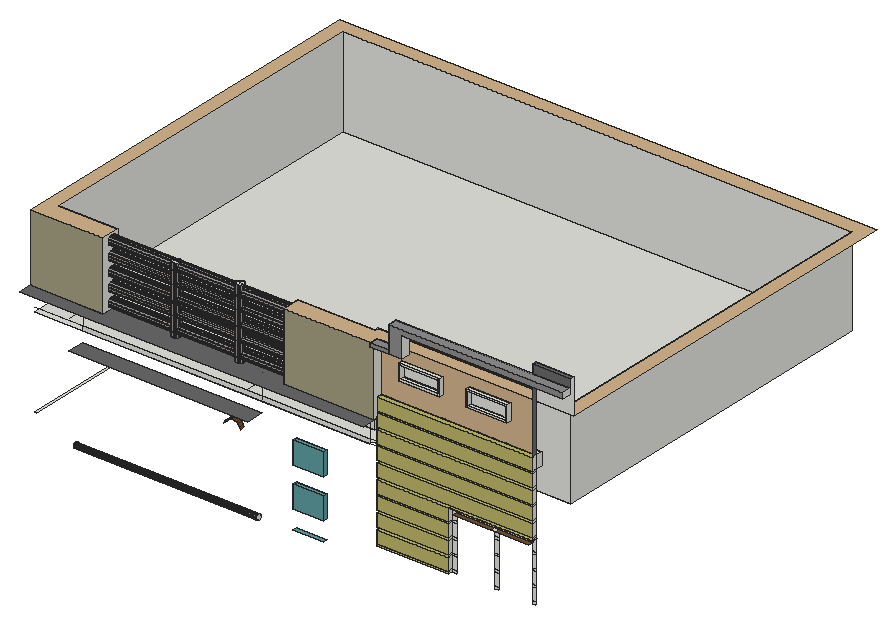
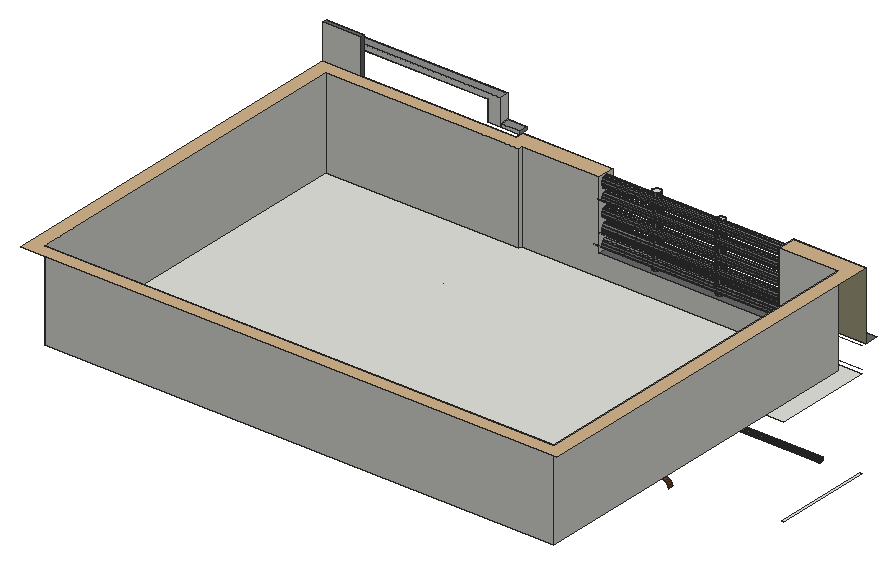
# SketchUp Ruby script. Lengths in inches.
U = 1.inch
M = Sketchup.active_model
def pt(a) = Geom::Point3d.new(a.map { |v| v * U })
def face(e, loops, mat)
  f = e.add_face(loops[0].map { |a| pt(a) })
  loops[1..].each { |l| e.add_face(l.map { |a| pt(a) }).erase! }
  f.material = f.back_material = mat if mat
  f
end
# faces: each face lists its corners as indices into pts; further lists are holes
def faces(e, pts, list, mat = nil) = list.each { |f| face(e, (f[0].is_a?(Array) ? f : [f]).map { |l| l.map { |i| pts[i] } }, mat) }
# xy, xz, yz: faces in a plane at the given z, y or x. An outline is a flat list of corners, or four numbers for a rectangle; further outlines are holes
def ring(l) = l.size == 4 ? [[l[0], l[1]], [l[2], l[1]], [l[2], l[3]], [l[0], l[3]]] : l.each_slice(2).to_a
def flat(e, list, mat, &to3) = list.each { |f| face(e, (f[0].is_a?(Array) ? f : [f]).map { |l| ring(l).map { |u, v| to3.(u, v) } }, mat) }
def xy(e, z, list, mat = nil) = flat(e, list, mat) { |x, y| [x, y, z] }
def xz(e, y, list, mat = nil) = flat(e, list, mat) { |x, z| [x, y, z] }
def yz(e, x, list, mat = nil) = flat(e, list, mat) { |y, z| [x, y, z] }
def lines(e, pts, list) = list.each { |a, b| e.add_line(pt(pts[a]), pt(pts[b])) }
# prism: a flat outline (further loops are holes) pulled along v
def prism(e, loops, v, mat = nil)
  f = face(e, loops, mat); d = Geom::Vector3d.new(v.map { |x| x * U })
  f.pushpull(f.normal.samedirection?(d) ? d.length : -d.length)
end
def box(e, o, s, mat = nil) = prism(e, [[o, [o[0] + s[0], o[1], o[2]], [o[0] + s[0], o[1] + s[1], o[2]], [o[0], o[1] + s[1], o[2]]]], [0, 0, s[2]], mat)
def at(x, y, z, deg = 0) = Geom::Transformation.translation(pt([x, y, z])) * Geom::Transformation.rotation(ORIGIN, Z_AXIS, deg.degrees)
def axes(o, x, y, z) = Geom::Transformation.new([*x, 0, *y, 0, *z, 0, *pt(o).to_a, 1])
def part(name) = M.definitions.add(name)
# library, detail: a bought-in or finely detailed component or shape, given as its bounding box
def library(name, o, s) = part(name).tap { |d| box(d.entities, o, s) }
def detail(e, o, s) = box(e.add_group.entities, o, s)
def put(e, d, t, mat = nil) = e.add_instance(d, t).tap { |i| i.material = mat if mat }
def group(e, t, mat = nil) = e.add_group.tap { |g| g.transformation = t; g.material = mat if mat }.entities
root = M.entities
M.materials.add("[0035_Tan]").color = [210, 180, 140]
M.materials.add("[0057_DarkKhaki]").color = [189, 183, 107]
M.materials.add("[0081_CadetBlue]").color = [95, 158, 160]
M.materials.add("[0134_DimGray]").color = [105, 105, 105]
M.materials.add("[Color M04]").color = [142, 142, 142]
M.materials.add("[Concrete Aggregate Smoke]").color = [154, 150, 148]
M.materials.add("[Sandstone]").color = [118, 81, 52]
M.materials.add("[Stone Coursed Rough]").color = [165, 160, 130]
M.materials.add("[Wood Veneer 01]").color = [120, 70, 37]
xy(root,183.125,[[0,109.375,1.6875,174.625]])
xy(root,183.41,[[230.5,108.71,278.53,111.71]],"[0057_DarkKhaki]")
xy(root,183.75,[[185.74,94.375,206.18,97.375]],"[0081_CadetBlue]")
xy(root,184.9375,[[230.5,108.71,278.53,111.71]],"[0057_DarkKhaki]")
xy(root,193.41,[[230.5,108.71,278.53,111.71]],"[0057_DarkKhaki]")
xy(root,194.9375,[[230.5,108.71,278.53,111.71]],"[0057_DarkKhaki]")
xy(root,196.125,[[185.74,94.375,206.18,97.375]],"[0081_CadetBlue]")
xy(root,203.41,[[230.5,108.71,278.53,111.71]],"[0057_DarkKhaki]")
xy(root,204,[[75.42,171.625,105.42,174.625]],"[Wood Veneer 01]")
xy(root,204.9375,[[230.5,108.71,278.53,111.71]],"[0057_DarkKhaki]")
xy(root,207,[[72.42,171.625,108.42,174.625]],"[Wood Veneer 01]")
xy(root,211.125,[[185.74,94.375,206.18,97.375]],"[0081_CadetBlue]")
xy(root,213.41,[[230.5,108.71,278.53,111.71]],"[0057_DarkKhaki]")
xy(root,214.9375,[[230.5,108.71,278.53,111.71]],"[0057_DarkKhaki]")
xy(root,220.14,[[307.0625,108.71,310.13,111.71]])
xy(root,220.14,[[281.53,108.71,307.0625,111.71],[310.13,108.71,332.6,111.71]],"[Sandstone]")
xy(root,222.6875,[[185.74,94.375,206.18,97.375]],"[0081_CadetBlue]")
xy(root,223.14,[[278.53,108.71,334.9375,111.71],[334.9375,108.71,335.6,111.71]])
xy(root,223.41,[[230.5,108.71,334.9375,111.71]],"[0057_DarkKhaki]")
xy(root,224.9375,[[230.5,108.71,334.9375,111.71]],"[0057_DarkKhaki]")
xy(root,233.41,[[230.5,108.71,334.9375,111.71]],"[0057_DarkKhaki]")
xy(root,234.9375,[[230.5,108.71,334.9375,111.71]],"[0057_DarkKhaki]")
xy(root,236.11,[[32.625,97.375,152.93,109.375]],"[0134_DimGray]")
xy(root,237.6875,[[185.74,94.375,206.18,97.375]],"[0081_CadetBlue]")
xy(root,243,[[0,109.375,0,174.625,228.875,174.625,228.875,111.71,225.1875,111.71,225.1875,109.375]])
xy(root,243.41,[[230.5,108.71,334.9375,111.71]],"[0057_DarkKhaki]")
xy(root,244.9375,[[230.5,108.71,334.9375,111.71]],"[0057_DarkKhaki]")
xy(root,246,[[9,118.375,221.5,118.375,221.5,120.71,351,120.71,351,357,9,357]])
xy(root,253.41,[[230.5,108.71,334.9375,111.71]],"[0057_DarkKhaki]")
xy(root,254.9375,[[230.5,108.71,334.9375,111.71]],"[0057_DarkKhaki]")
xy(root,260.3125,[[32.625,106.375,48.47,109.375],[169.54,106.375,225.1875,109.375],[225.1875,106.375,230.5,109.375],[93.22,109.28,93.6,109.375,92.22,109.375,92.51,109.29]])
xy(root,260.3125,[[[0,97.375,230.5,97.375,230.5,106.375,169.54,106.375,169.54,118.375,48.47,118.375,48.47,106.375,0,106.375],[93.22,109.28,92.51,109.29,92.22,109.375,91.82,109.49,91.2,109.86,90.7,110.38,90.35,111.01,90.18,111.7,90.19,112.42,90.39,113.11,90.76,113.73,91.28,114.22,91.91,114.57,92.6,114.75,93.32,114.73,94.01,114.53,94.625,114.16,95.125,113.65,95.47,113.02,95.65,112.32,95.63,111.61,95.43,110.92,95.06,110.3,94.55,109.8,93.92,109.45,93.6,109.375],[135.16,109.375,134.75,109.49,134.14,109.86,133.64,110.38,133.29,111.01,133.12,111.7,133.13,112.42,133.33,113.11,133.7,113.73,134.22,114.22,134.84,114.57,135.54,114.75,136.26,114.73,136.95,114.53,137.5625,114.16,138.0625,113.65,138.41,113.02,138.58,112.32,138.57,111.61,138.37,110.92,138,110.3,137.49,109.8,136.86,109.45,136.54,109.375]]],"[0134_DimGray]")
xy(root,263.41,[[230.5,108.71,334.9375,111.71]],"[0057_DarkKhaki]")
xy(root,264.9375,[[230.5,111.71,334.9375,116.15]])
xy(root,264.9375,[[230.5,108.71,334.9375,111.71]],"[0057_DarkKhaki]")
xy(root,273.41,[[230.5,111.71,334.9375,116.15]])
xy(root,273.41,[[230.5,108.71,334.9375,111.71]],"[0057_DarkKhaki]")
xy(root,288.05,[[245,108.71,272.5625,111.71],[290.25,108.71,317.8125,111.71]])
xy(root,288.97,[[291.17,108.71,316.89,111.71]])
xy(root,289.17,[[246.12,108.71,271.44,111.71]])
xy(root,297.62,[[246.12,108.71,271.44,111.71]])
xy(root,297.82,[[291.17,108.71,316.89,111.71]])
xy(root,298.74,[[245,108.71,272.5625,111.71],[290.25,108.71,317.8125,111.71]])
xy(root,305.12,[[92.22,109.375,93.6,109.375,93.92,109.45,94.55,109.8,95.06,110.3,95.43,110.92,95.63,111.61,95.65,112.32,95.63,112.38,90.19,112.38,90.18,111.7,90.35,111.01,90.7,110.38,91.2,109.86,91.82,109.49],[90.19,112.38,95.63,112.38,95.47,113.02,95.125,113.65,94.72,114.07,91.11,114.07,90.76,113.73,90.39,113.11,90.19,112.42],[91.11,114.07,94.72,114.07,94.625,114.16,94.01,114.53,93.32,114.73,92.6,114.75,91.91,114.57,91.28,114.22]])
xy(root,306,[[230.5,102.71,243,108.71],[243,102.71,251.83,108.71]])
xy(root,306,[[0,106.375,48.47,106.375,48.47,118.375,9,118.375,9,357,351,357,351,120.71,221.5,120.71,221.5,118.375,169.54,118.375,169.54,106.375,230.5,106.375,230.5,111.71,360,111.71,360,366,0,366]],"[0035_Tan]")
xy(root,306.9375,[[135.16,109.375,136.54,109.375,136.86,109.45,137.49,109.8,138,110.3,138.37,110.92,138.57,111.61,138.58,112.32,138.41,113.02,138.0625,113.65,137.5625,114.16,136.95,114.53,136.26,114.73,135.54,114.75,134.84,114.57,134.22,114.22,133.7,113.73,133.33,113.11,133.13,112.42,133.12,111.7,133.29,111.01,133.64,110.38,134.14,109.86,134.75,109.49]])
xy(root,308.21,[[230.5,102.71,243,108.71]],"[Color M04]")
xy(root,320.08,[[251.83,102.71,360,108.71]])
xy(root,323.78,[[243,102.71,360,108.71]],"[Color M04]")
xy(root,329.5,[[334.9375,108.71,360,111.71]],"[0134_DimGray]")
xz(root,94.375,[[185.74,196.125,206.18,211.125],[185.74,222.6875,206.18,237.6875]],"[0081_CadetBlue]")
xz(root,97.375,[[185.74,196.125,206.18,211.125],[185.74,222.6875,206.18,237.6875]])
xz(root,102.71,[[230.5,306,243,308.21],[243,306,251.83,306,251.83,320.08,360,320.08,360,323.78,243,323.78]],"[Color M04]")
xz(root,106.375,[[0,260.3125,48.47,306],[169.54,260.3125,230.5,306]],"[Stone Coursed Rough]")
xz(root,108.71,[[[245,288.05,272.5625,298.74],[246.12,289.17,271.44,297.62]],[[290.25,288.05,317.8125,298.74],[291.17,288.97,316.89,297.82]],[230.5,306,243,308.21],[243,306,243,323.78,334.9375,323.78,334.9375,320.08,251.83,320.08,251.83,306],[334.9375,320.08,360,323.78]])
xz(root,108.71,[[230.5,184.9375,278.53,193.41],[230.5,194.9375,278.53,203.41],[230.5,204.9375,278.53,213.41],[230.5,214.9375,278.53,214.9375,278.53,223.14,334.9375,223.14,334.9375,223.41,230.5,223.41],[230.5,224.9375,334.9375,233.41],
  [230.5,234.9375,334.9375,243.41],[230.5,244.9375,334.9375,253.41],[230.5,254.9375,334.9375,263.41],[230.5,264.9375,334.9375,273.41]],"[0057_DarkKhaki]")
xz(root,108.71,[[334.9375,323.78,360,329.5]],"[0134_DimGray]")
xz(root,109.375,[[32.625,243,152.93,246],[152.93,243,225.1875,246]])
xz(root,109.375,[[92.22,260.3125,93.6,305.12],[135.16,260.3125,136.54,306.9375]],"[Concrete Aggregate Smoke]")
xz(root,111.71,[[230.5,183.41,278.53,184.9375],[278.53,183.41,281.53,184.9375],[307.0625,183.41,310.13,184.9375],[332.6,183.41,334.9375,184.9375],[230.5,184.9375,278.53,193.41],
  [278.53,184.9375,281.53,193.41],[307.0625,184.9375,310.13,193.41],[332.6,184.9375,334.9375,193.41],[230.5,193.41,278.53,194.9375],[278.53,193.41,281.53,194.9375],
  [307.0625,193.41,310.13,194.9375],[332.6,193.41,334.9375,194.9375],[230.5,194.9375,278.53,203.41],[278.53,194.9375,281.53,203.41],[307.0625,194.9375,310.13,203.41],
  [332.6,194.9375,334.9375,203.41],[230.5,203.41,278.53,204.9375],[278.53,203.41,281.53,204.9375],[307.0625,203.41,310.13,204.9375],[332.6,203.41,334.9375,204.9375],
  [230.5,204.9375,278.53,213.41],[278.53,204.9375,281.53,213.41],[307.0625,204.9375,310.13,213.41],[332.6,204.9375,334.9375,213.41],[230.5,213.41,278.53,214.9375],
  [278.53,213.41,281.53,214.9375],[307.0625,213.41,310.13,214.9375],[332.6,213.41,334.9375,214.9375],[230.5,214.9375,230.5,223.41,334.9375,223.41,334.9375,223.14,278.53,223.14,278.53,214.9375],[278.53,214.9375,281.53,214.9375,281.53,220.14,332.6,220.14,332.6,214.9375,334.9375,214.9375,334.9375,223.14,278.53,223.14],
  [307.0625,214.9375,310.13,220.14],[230.5,224.9375,334.9375,233.41],[230.5,234.9375,334.9375,243.41],[230.5,244.9375,334.9375,253.41],[230.5,254.9375,334.9375,263.41],
  [230.5,264.9375,334.9375,273.41],[[245,288.05,272.5625,298.74],[246.12,289.17,271.44,297.62]],[[290.25,288.05,317.8125,298.74],[291.17,288.97,316.89,297.82]],[291.17,288.97,316.89,297.82],[246.12,289.17,271.44,297.62],
  [334.9375,306,360,329.5]])
xz(root,111.71,[[[230.5,273.41,334.9375,306],[245,288.05,272.5625,298.74],[290.25,288.05,317.8125,298.74]]],"[0035_Tan]")
xz(root,111.71,[[230.5,223.41,334.9375,224.9375],[230.5,233.41,334.9375,234.9375],[230.5,243.41,334.9375,244.9375],[230.5,253.41,334.9375,254.9375],[230.5,263.41,334.9375,264.9375]],"[0057_DarkKhaki]")
xz(root,116.15,[[230.5,264.9375,334.9375,273.41]])
xz(root,118.375,[[9,246,9,306,48.47,306,48.47,260.3125,169.54,260.3125,169.54,306,221.5,306,221.5,246]])
xz(root,120.71,[[221.5,246,351,306]])
xz(root,357,[[9,246,351,306]])
yz(root,9,[[118.375,246,357,306]])
yz(root,48.47,[[[106.375,260.3125,118.375,306],[113.22,298.73,112.38,298.84,111.6,299.17,110.93,299.68,110.41,300.35,110.08,301.14,109.97,301.98,110.08,302.82,110.41,303.6,110.93,304.28,111.6,304.79,112.38,305.12,113.22,305.23,114.07,305.12,114.85,304.79,115.52,304.28,116.04,303.6,116.36,302.82,116.47,301.98,116.36,301.14,116.04,300.35,115.52,299.68,114.85,299.17,114.07,298.84],[113.22,289.42,112.38,289.53,111.6,289.85,110.93,290.37,110.41,291.04,110.08,291.83,109.97,292.67,110.08,293.51,110.41,294.29,110.93,294.97,111.6,295.48,112.38,295.81,113.22,295.92,114.07,295.81,114.85,295.48,115.52,294.97,116.04,294.29,116.36,293.51,116.47,292.67,116.36,291.83,116.04,291.04,115.52,290.37,114.85,289.85,114.07,289.53],[113.22,280.1,112.38,280.22,111.6,280.54,110.93,281.06,110.41,281.73,110.08,282.51,109.97,283.35,110.08,284.2,110.41,284.98,110.93,285.65,111.6,286.17,112.38,286.49,113.22,286.6,114.07,286.49,114.85,286.17,115.52,285.65,116.04,284.98,116.36,284.2,116.47,283.35,116.36,282.51,116.04,281.73,115.52,281.06,114.85,280.54,114.07,280.22],[113.22,270.79,112.38,270.9,111.6,271.23,110.93,271.74,110.41,272.42,110.08,273.2,109.97,274.04,110.08,274.88,110.41,275.67,110.93,276.34,111.6,276.86,112.38,277.18,113.22,277.29,114.07,277.18,114.85,276.86,115.52,276.34,116.04,275.67,116.36,274.88,116.47,274.04,116.36,273.2,116.04,272.42,115.52,271.74,114.85,271.23,114.07,270.9],[113.22,261.48,112.38,261.59,111.6,261.92,110.93,262.43,110.41,263.1,110.08,263.89,109.97,264.73,110.08,265.57,110.41,266.35,110.93,267.03,111.6,267.54,112.38,267.87,113.22,267.98,114.07,267.87,114.85,267.54,115.52,267.03,116.04,266.35,116.36,265.57,116.47,264.73,116.36,263.89,116.04,263.1,115.52,262.43,114.85,261.92,114.07,261.59]]])
yz(root,155.875,[[102.77,175.55,103.19,175.61,103.58,175.77,103.92,176.03,104.18,176.37,104.34,176.76,104.4,177.18,104.34,177.6,104.18,177.99,103.92,178.33,103.58,178.59,103.19,178.75,102.77,178.8,102.35,178.75,101.96,178.59,101.62,178.33,101.36,177.99,101.2,177.6,101.15,177.18,101.2,176.76,101.36,176.37,101.62,176.03,101.96,175.77,102.35,175.61]])
yz(root,169.54,[[[106.375,260.3125,118.375,306],[113.22,298.73,114.07,298.84,114.85,299.17,115.52,299.68,116.04,300.35,116.36,301.14,116.47,301.98,116.36,302.82,116.04,303.6,115.52,304.28,114.85,304.79,114.07,305.12,113.22,305.23,112.38,305.12,111.6,304.79,110.93,304.28,110.41,303.6,110.08,302.82,109.97,301.98,110.08,301.14,110.41,300.35,110.93,299.68,111.6,299.17,112.38,298.84],[113.22,280.1,114.07,280.22,114.85,280.54,115.52,281.06,116.04,281.73,116.36,282.51,116.47,283.35,116.36,284.2,116.04,284.98,115.52,285.65,114.85,286.17,114.07,286.49,113.22,286.6,112.38,286.49,111.6,286.17,110.93,285.65,110.41,284.98,110.08,284.2,109.97,283.35,110.08,282.51,110.41,281.73,110.93,281.06,111.6,280.54,112.38,280.22],[113.22,270.79,114.07,270.9,114.85,271.23,115.52,271.74,116.04,272.42,116.36,273.2,116.47,274.04,116.36,274.88,116.04,275.67,115.52,276.34,114.85,276.86,114.07,277.18,113.22,277.29,112.38,277.18,111.6,276.86,110.93,276.34,110.41,275.67,110.08,274.88,109.97,274.04,110.08,273.2,110.41,272.42,110.93,271.74,111.6,271.23,112.38,270.9]]])
yz(root,172.59,[[113.22,289.42,114.07,289.53,114.85,289.85,115.52,290.37,116.04,291.04,116.36,291.83,116.47,292.67,116.36,293.51,116.04,294.29,115.52,294.97,114.85,295.48,114.07,295.81,113.22,295.92,112.38,295.81,111.6,295.48,110.93,294.97,110.41,294.29,110.08,293.51,109.97,292.67,110.08,291.83,110.41,291.04,110.93,290.37,111.6,289.85,112.38,289.53]])
yz(root,175.03,[[113.22,261.48,114.07,261.59,114.85,261.92,115.52,262.43,116.04,263.1,116.36,263.89,116.47,264.73,116.36,265.57,116.04,266.35,115.52,267.03,114.85,267.54,114.07,267.87,113.22,267.98,112.38,267.87,111.6,267.54,110.93,267.03,110.41,266.35,110.08,265.57,109.97,264.73,110.08,263.89,110.41,263.1,110.93,262.43,111.6,261.92,112.38,261.59]])
yz(root,185.74,[[94.375,196.125,97.375,211.125],[94.375,222.6875,97.375,237.6875]],"[0081_CadetBlue]")
yz(root,206.18,[[94.375,196.125,97.375,211.125],[94.375,222.6875,97.375,237.6875]],"[0081_CadetBlue]")
yz(root,221.5,[[118.375,246,120.71,306]])
yz(root,230.5,[[108.71,184.9375,111.71,193.41],[108.71,194.9375,111.71,203.41],[108.71,204.9375,111.71,213.41],[108.71,214.9375,111.71,223.41],[108.71,224.9375,111.71,233.41],
  [108.71,234.9375,111.71,243],[108.71,243,111.71,243.41],[108.71,244.9375,111.71,253.41],[108.71,254.9375,111.71,263.41],[106.375,260.3125,108.71,260.3125,108.71,263.41,111.71,263.41,111.71,264.9375,108.71,264.9375,108.71,273.41,111.71,273.41,111.71,306,106.375,306],
  [108.71,264.9375,111.71,273.41],[111.71,264.9375,116.15,273.41]])
yz(root,230.5,[[102.71,306,108.71,308.21]],"[Color M04]")
yz(root,243,[[102.71,306,108.71,308.21],[102.71,308.21,108.71,323.78]])
yz(root,245,[[108.71,288.05,111.71,298.74]])
yz(root,246.12,[[108.71,289.17,111.71,297.62]])
yz(root,251.83,[[102.71,306,108.71,320.08]])
yz(root,271.44,[[108.71,289.17,111.71,297.62]])
yz(root,272.5625,[[108.71,288.05,111.71,298.74]])
yz(root,278.53,[[108.71,183.41,111.71,184.9375],[108.71,184.9375,111.71,193.41],[108.71,193.41,111.71,194.9375],[108.71,194.9375,111.71,203.41],[108.71,203.41,111.71,204.9375],
  [108.71,204.9375,111.71,213.41],[108.71,213.41,111.71,214.9375],[108.71,214.9375,111.71,223.14]])
yz(root,290.25,[[108.71,288.05,111.71,298.74]])
yz(root,291.17,[[108.71,288.97,111.71,297.82]])
yz(root,316.89,[[108.71,288.97,111.71,297.82]])
yz(root,317.8125,[[108.71,288.05,111.71,298.74]])
yz(root,334.9375,[[108.71,223.14,111.71,223.41],[108.71,223.41,111.71,224.9375],[108.71,224.9375,111.71,233.41],[108.71,233.41,111.71,234.9375],[108.71,234.9375,111.71,243.41],
  [108.71,243.41,111.71,244.9375],[108.71,244.9375,111.71,253.41],[108.71,253.41,111.71,254.9375],[108.71,254.9375,111.71,263.41],[108.71,263.41,111.71,264.9375],
  [108.71,264.9375,111.71,273.41],[111.71,264.9375,116.15,273.41]])
yz(root,334.9375,[[108.71,273.41,111.71,329.5]],"[0134_DimGray]")
yz(root,351,[[120.71,246,357,306]])
yz(root,360,[[102.71,320.08,108.71,323.78]])
p = [[32.625,101.96,175.77],[32.625,102.35,175.61],[155.875,102.35,175.61],[155.875,101.96,175.77],[32.625,102.77,175.55],[155.875,102.77,175.55],
  [32.625,103.19,175.61],[155.875,103.19,175.61],[32.625,103.58,175.77],[155.875,103.58,175.77],[32.625,101.62,176.03],[155.875,101.62,176.03],
  [32.625,103.92,176.03],[155.875,103.92,176.03],[77.94,174.625,177.23],[77.39,174.625,175.83],[77.39,171.625,175.83],[77.94,171.625,177.23],
  [32.625,101.36,176.37],[155.875,101.36,176.37],[32.625,104.18,176.37],[155.875,104.18,176.37],[88.5,174.625,176.02],[87.9,174.625,177.39],
  [87.9,171.625,177.39],[88.5,171.625,176.02],[32.625,101.2,176.76],[155.875,101.2,176.76],[32.625,104.34,176.76],[155.875,104.34,176.76],
  [32.625,101.15,177.18],[155.875,101.15,177.18],[32.625,104.4,177.18],[155.875,104.4,177.18],[32.625,101.2,177.6],[155.875,101.2,177.6],
  [32.625,104.34,177.6],[155.875,104.34,177.6],[78.84,174.625,178.4375],[78.84,171.625,178.4375],[86.97,174.625,178.57],[86.97,171.625,178.57],
  [32.625,101.36,177.99],[155.875,101.36,177.99],[32.625,104.18,177.99],[155.875,104.18,177.99],[32.625,101.62,178.33],[155.875,101.62,178.33],
  [32.625,103.92,178.33],[155.875,103.92,178.33],[32.625,101.96,178.59],[155.875,101.96,178.59],[32.625,103.58,178.59],[155.875,103.58,178.59],
  [80.01,174.625,179.37],[80.01,171.625,179.37],[32.625,102.35,178.75],[155.875,102.35,178.75],[32.625,103.19,178.75],[155.875,103.19,178.75],
  [85.76,174.625,179.46],[85.76,171.625,179.46],[32.625,102.77,178.8],[155.875,102.77,178.8],[81.39,174.625,179.97],[81.39,171.625,179.97],
  [84.37,174.625,180.02],[84.37,171.625,180.02],[82.875,174.625,180.1875],[82.875,171.625,180.1875],[91.82,109.49,260.3125],[92.22,109.375,260.3125],
  [92.22,109.375,305.12],[91.82,109.49,305.12],[93.6,109.375,260.3125],[93.92,109.45,260.3125],[93.92,109.45,305.12],[93.6,109.375,305.12],
  [134.75,109.49,260.3125],[135.16,109.375,260.3125],[135.16,109.375,306.9375],[134.75,109.49,306.9375],[136.54,109.375,260.3125],[136.86,109.45,260.3125],
  [136.86,109.45,306.9375],[136.54,109.375,306.9375],[91.2,109.86,260.3125],[91.2,109.86,305.12],[94.55,109.8,260.3125],[94.55,109.8,305.12],
  [134.14,109.86,260.3125],[134.14,109.86,306.9375],[137.49,109.8,260.3125],[137.49,109.8,306.9375],[95.06,110.3,260.3125],[95.06,110.3,305.12],
  [138,110.3,260.3125],[138,110.3,306.9375],[90.7,110.38,260.3125],[90.7,110.38,305.12],[133.64,110.38,260.3125],[133.64,110.38,306.9375],
  [95.43,110.92,260.3125],[95.43,110.92,305.12],[138.37,110.92,260.3125],[138.37,110.92,306.9375],[90.35,111.01,260.3125],[90.35,111.01,305.12],
  [133.29,111.01,260.3125],[133.29,111.01,306.9375],[95.63,111.61,260.3125],[95.63,111.61,305.12],[138.57,111.61,260.3125],[138.57,111.61,306.9375],
  [90.18,111.7,260.3125],[90.18,111.7,305.12],[133.12,111.7,260.3125],[133.12,111.7,306.9375],[95.65,112.32,260.3125],[95.65,112.32,305.12],
  [138.58,112.32,260.3125],[138.58,112.32,306.9375],[90.19,112.42,260.3125],[90.19,112.38,305.12],[90.19,112.42,305.12],[133.13,112.42,260.3125],
  [133.13,112.42,306.9375],[95.47,113.02,260.3125],[95.47,113.02,305.12],[95.63,112.38,305.12],[138.41,113.02,260.3125],[138.41,113.02,306.9375],
  [90.39,113.11,260.3125],[90.39,113.11,305.12],[133.33,113.11,260.3125],[133.33,113.11,306.9375],[95.125,113.65,260.3125],[95.125,113.65,305.12],
  [138.0625,113.65,260.3125],[138.0625,113.65,306.9375],[90.76,113.73,260.3125],[90.76,113.73,305.12],[133.7,113.73,260.3125],[133.7,113.73,306.9375],
  [94.625,114.16,260.3125],[94.625,114.16,305.12],[94.72,114.07,305.12],[137.5625,114.16,260.3125],[137.5625,114.16,306.9375],[91.28,114.22,260.3125],
  [91.11,114.07,305.12],[91.28,114.22,305.12],[134.22,114.22,260.3125],[134.22,114.22,306.9375],[91.91,114.57,260.3125],[91.91,114.57,305.12],
  [94.01,114.53,260.3125],[94.01,114.53,305.12],[134.84,114.57,260.3125],[134.84,114.57,306.9375],[136.95,114.53,260.3125],[136.95,114.53,306.9375],
  [93.32,114.73,260.3125],[93.32,114.73,305.12],[136.26,114.73,260.3125],[136.26,114.73,306.9375],[92.6,114.75,260.3125],[92.6,114.75,305.12],
  [135.54,114.75,260.3125],[135.54,114.75,306.9375],[48.47,112.38,261.59],[48.47,113.22,261.48],[175.03,113.22,261.48],[175.03,112.38,261.59],
  [48.47,114.07,261.59],[175.03,114.07,261.59],[48.47,111.6,261.92],[175.03,111.6,261.92],[48.47,114.85,261.92],[175.03,114.85,261.92],
  [48.47,110.93,262.43],[175.03,110.93,262.43],[48.47,115.52,262.43],[175.03,115.52,262.43],[48.47,110.41,263.1],[175.03,110.41,263.1],
  [48.47,116.04,263.1],[175.03,116.04,263.1],[48.47,110.08,263.89],[175.03,110.08,263.89],[48.47,116.36,263.89],[175.03,116.36,263.89],
  [48.47,109.97,264.73],[175.03,109.97,264.73],[48.47,116.47,264.73],[175.03,116.47,264.73],[48.47,110.08,265.57],[175.03,110.08,265.57],
  [48.47,116.36,265.57],[175.03,116.36,265.57],[48.47,110.41,266.35],[175.03,110.41,266.35],[48.47,116.04,266.35],[175.03,116.04,266.35],
  [48.47,110.93,267.03],[175.03,110.93,267.03],[48.47,115.52,267.03],[175.03,115.52,267.03],[48.47,111.6,267.54],[175.03,111.6,267.54],
  [48.47,114.85,267.54],[175.03,114.85,267.54],[48.47,112.38,267.87],[175.03,112.38,267.87],[48.47,114.07,267.87],[175.03,114.07,267.87],
  [48.47,113.22,267.98],[175.03,113.22,267.98],[48.47,112.38,270.9],[48.47,113.22,270.79],[169.54,113.22,270.79],[169.54,112.38,270.9],
  [48.47,114.07,270.9],[169.54,114.07,270.9],[48.47,111.6,271.23],[169.54,111.6,271.23],[48.47,114.85,271.23],[169.54,114.85,271.23],
  [48.47,110.93,271.74],[169.54,110.93,271.74],[48.47,115.52,271.74],[169.54,115.52,271.74],[48.47,110.41,272.42],[169.54,110.41,272.42],
  [48.47,116.04,272.42],[169.54,116.04,272.42],[48.47,110.08,273.2],[169.54,110.08,273.2],[48.47,116.36,273.2],[169.54,116.36,273.2],
  [48.47,109.97,274.04],[169.54,109.97,274.04],[48.47,116.47,274.04],[169.54,116.47,274.04],[48.47,110.08,274.88],[169.54,110.08,274.88],
  [48.47,116.36,274.88],[169.54,116.36,274.88],[48.47,110.41,275.67],[169.54,110.41,275.67],[48.47,116.04,275.67],[169.54,116.04,275.67],
  [48.47,110.93,276.34],[169.54,110.93,276.34],[48.47,115.52,276.34],[169.54,115.52,276.34],[48.47,111.6,276.86],[169.54,111.6,276.86],
  [48.47,114.85,276.86],[169.54,114.85,276.86],[48.47,112.38,277.18],[169.54,112.38,277.18],[48.47,114.07,277.18],[169.54,114.07,277.18],
  [48.47,113.22,277.29],[169.54,113.22,277.29],[48.47,112.38,280.22],[48.47,113.22,280.1],[169.54,113.22,280.1],[169.54,112.38,280.22],
  [48.47,114.07,280.22],[169.54,114.07,280.22],[48.47,111.6,280.54],[169.54,111.6,280.54],[48.47,114.85,280.54],[169.54,114.85,280.54],
  [48.47,110.93,281.06],[169.54,110.93,281.06],[48.47,115.52,281.06],[169.54,115.52,281.06],[48.47,110.41,281.73],[169.54,110.41,281.73],
  [48.47,116.04,281.73],[169.54,116.04,281.73],[48.47,110.08,282.51],[169.54,110.08,282.51],[48.47,116.36,282.51],[169.54,116.36,282.51],
  [48.47,109.97,283.35],[169.54,109.97,283.35],[48.47,116.47,283.35],[169.54,116.47,283.35],[48.47,110.08,284.2],[169.54,110.08,284.2],
  [48.47,116.36,284.2],[169.54,116.36,284.2],[48.47,110.41,284.98],[169.54,110.41,284.98],[48.47,116.04,284.98],[169.54,116.04,284.98],
  [48.47,110.93,285.65],[169.54,110.93,285.65],[48.47,115.52,285.65],[169.54,115.52,285.65],[48.47,111.6,286.17],[169.54,111.6,286.17],
  [48.47,114.85,286.17],[169.54,114.85,286.17],[48.47,112.38,286.49],[169.54,112.38,286.49],[48.47,114.07,286.49],[169.54,114.07,286.49],
  [48.47,113.22,286.6],[169.54,113.22,286.6],[48.47,112.38,289.53],[48.47,113.22,289.42],[172.59,113.22,289.42],[172.59,112.38,289.53],
  [48.47,114.07,289.53],[172.59,114.07,289.53],[48.47,111.6,289.85],[172.59,111.6,289.85],[48.47,114.85,289.85],[172.59,114.85,289.85],
  [48.47,110.93,290.37],[172.59,110.93,290.37],[48.47,115.52,290.37],[172.59,115.52,290.37],[48.47,110.41,291.04],[172.59,110.41,291.04],
  [48.47,116.04,291.04],[172.59,116.04,291.04],[48.47,110.08,291.83],[172.59,110.08,291.83],[48.47,116.36,291.83],[172.59,116.36,291.83],
  [48.47,109.97,292.67],[172.59,109.97,292.67],[48.47,116.47,292.67],[172.59,116.47,292.67],[48.47,110.08,293.51],[172.59,110.08,293.51],
  [48.47,116.36,293.51],[172.59,116.36,293.51],[48.47,110.41,294.29],[172.59,110.41,294.29],[48.47,116.04,294.29],[172.59,116.04,294.29],
  [48.47,110.93,294.97],[172.59,110.93,294.97],[48.47,115.52,294.97],[172.59,115.52,294.97],[48.47,111.6,295.48],[172.59,111.6,295.48],
  [48.47,114.85,295.48],[172.59,114.85,295.48],[48.47,112.38,295.81],[172.59,112.38,295.81],[48.47,114.07,295.81],[172.59,114.07,295.81],
  [48.47,113.22,295.92],[172.59,113.22,295.92],[48.47,112.38,298.84],[48.47,113.22,298.73],[169.54,113.22,298.73],[169.54,112.38,298.84],
  [48.47,114.07,298.84],[169.54,114.07,298.84],[48.47,111.6,299.17],[169.54,111.6,299.17],[48.47,114.85,299.17],[169.54,114.85,299.17],
  [48.47,110.93,299.68],[169.54,110.93,299.68],[48.47,115.52,299.68],[169.54,115.52,299.68],[48.47,110.41,300.35],[169.54,110.41,300.35],
  [48.47,116.04,300.35],[169.54,116.04,300.35],[48.47,110.08,301.14],[169.54,110.08,301.14],[48.47,116.36,301.14],[169.54,116.36,301.14],
  [48.47,109.97,301.98],[169.54,109.97,301.98],[48.47,116.47,301.98],[169.54,116.47,301.98],[48.47,110.08,302.82],[169.54,110.08,302.82],
  [48.47,116.36,302.82],[169.54,116.36,302.82],[48.47,110.41,303.6],[169.54,110.41,303.6],[48.47,116.04,303.6],[169.54,116.04,303.6],
  [48.47,110.93,304.28],[169.54,110.93,304.28],[48.47,115.52,304.28],[169.54,115.52,304.28],[48.47,111.6,304.79],[169.54,111.6,304.79],
  [48.47,114.85,304.79],[169.54,114.85,304.79],[48.47,112.38,305.12],[169.54,112.38,305.12],[48.47,114.07,305.12],[169.54,114.07,305.12],
  [48.47,113.22,305.23],[169.54,113.22,305.23],[152.93,97.375,255.79],[152.93,109.375,255.79],[228.875,174.625,243],[228.875,174.625,246],
  [225.1875,109.375,243],[230.5,109.375,243],[32.625,97.375,255.79],[32.625,109.375,255.79],[225.1875,109.375,246],[230.5,109.375,246],
  [0,109.375,246],[32.625,109.375,246],[225.1875,109.375,260.3125],[152.93,109.375,246],[32.625,109.375,260.3125],[152.93,109.375,260.3125],
  [0,109.375,260.3125]]
faces(root,p,[[0,1,2,3],[1,4,5,2],[4,6,7,5],[6,8,9,7],[10,0,3,11],[8,12,13,9],[18,10,11,19],[12,20,21,13],
  [26,18,19,27],[20,28,29,21],[30,26,27,31],[28,32,33,29],[34,30,31,35],[32,36,37,33],[42,34,35,43],[36,44,45,37],
  [46,42,43,47],[44,48,49,45],[50,46,47,51],[48,52,53,49],[56,50,51,57],[52,58,59,53],[62,56,57,63],[58,62,63,59],
  [70,71,72,73],[74,75,76,77],[78,79,80,81],[82,83,84,85],[86,70,73,87],[75,88,89,76],[90,78,81,91],[83,92,93,84],
  [88,94,95,89],[92,96,97,93],[98,86,87,99],[100,90,91,101],[94,102,103,95],[96,104,105,97],[106,98,99,107],[108,100,101,109],
  [102,110,111,103],[104,112,113,105],[114,106,107,115],[116,108,109,117],[110,118,119,111],[112,120,121,113],[122,114,115,123,124],[125,116,117,126],
  [118,127,128,129,119],[120,130,131,121],[132,122,124,133],[134,125,126,135],[127,136,137,128],[130,138,139,131],[140,132,133,141],[142,134,135,143],
  [136,144,145,146,137],[138,147,148,139],[149,140,141,150,151],[152,142,143,153],[154,149,151,155],[144,156,157,145],[158,152,153,159],[147,160,161,148],
  [156,162,163,157],[160,164,165,161],[166,154,155,167],[168,158,159,169],[162,166,167,163],[164,168,169,165],[170,171,172,173],[171,174,175,172],
  [176,170,173,177],[174,178,179,175],[180,176,177,181],[178,182,183,179],[184,180,181,185],[182,186,187,183],[188,184,185,189],[186,190,191,187],
  [192,188,189,193],[190,194,195,191],[196,192,193,197],[194,198,199,195],[200,196,197,201],[198,202,203,199],[204,200,201,205],[202,206,207,203],
  [208,204,205,209],[206,210,211,207],[212,208,209,213],[210,214,215,211],[216,212,213,217],[214,216,217,215],[218,219,220,221],[219,222,223,220],
  [224,218,221,225],[222,226,227,223],[228,224,225,229],[226,230,231,227],[232,228,229,233],[230,234,235,231],[236,232,233,237],[234,238,239,235],
  [240,236,237,241],[238,242,243,239],[244,240,241,245],[242,246,247,243],[248,244,245,249],[246,250,251,247],[252,248,249,253],[250,254,255,251],
  [256,252,253,257],[254,258,259,255],[260,256,257,261],[258,262,263,259],[264,260,261,265],[262,264,265,263],[266,267,268,269],[267,270,271,268],
  [272,266,269,273],[270,274,275,271],[276,272,273,277],[274,278,279,275],[280,276,277,281],[278,282,283,279],[284,280,281,285],[282,286,287,283],
  [288,284,285,289],[286,290,291,287],[292,288,289,293],[290,294,295,291],[296,292,293,297],[294,298,299,295],[300,296,297,301],[298,302,303,299],
  [304,300,301,305],[302,306,307,303],[308,304,305,309],[306,310,311,307],[312,308,309,313],[310,312,313,311],[314,315,316,317],[315,318,319,316],
  [320,314,317,321],[318,322,323,319],[324,320,321,325],[322,326,327,323],[328,324,325,329],[326,330,331,327],[332,328,329,333],[330,334,335,331],
  [336,332,333,337],[334,338,339,335],[340,336,337,341],[338,342,343,339],[344,340,341,345],[342,346,347,343],[348,344,345,349],[346,350,351,347],
  [352,348,349,353],[350,354,355,351],[356,352,353,357],[354,358,359,355],[360,356,357,361],[358,360,361,359],[362,363,364,365],[363,366,367,364],
  [368,362,365,369],[366,370,371,367],[372,368,369,373],[370,374,375,371],[376,372,373,377],[374,378,379,375],[380,376,377,381],[378,382,383,379],
  [384,380,381,385],[382,386,387,383],[388,384,385,389],[386,390,391,387],[392,388,389,393],[390,394,395,391],[396,392,393,397],[394,398,399,395],
  [400,396,397,401],[398,402,403,399],[404,400,401,405,129,123],[402,406,150,146,407,403],[408,404,123,129,405,409],[406,408,409,407,146,150]],"[Concrete Aggregate Smoke]")
faces(root,p,[[14,15,16,17],[22,23,24,25],[38,14,17,39],[23,40,41,24],[54,38,39,55],[40,60,61,41],[64,54,55,65],[60,66,67,61],
  [68,64,65,69],[66,68,69,67]],"[Wood Veneer 01]")
lines(root,p,[[410,411],[412,413],[414,415],[416,417],[418,419],[420,421],[418,422],[421,417],[423,411],[417,424],[411,425],[424,426]])
